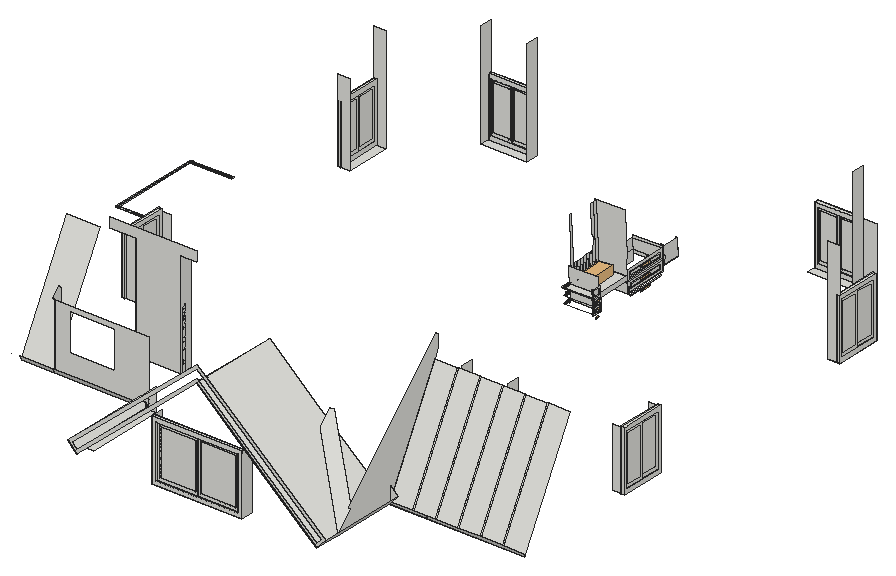
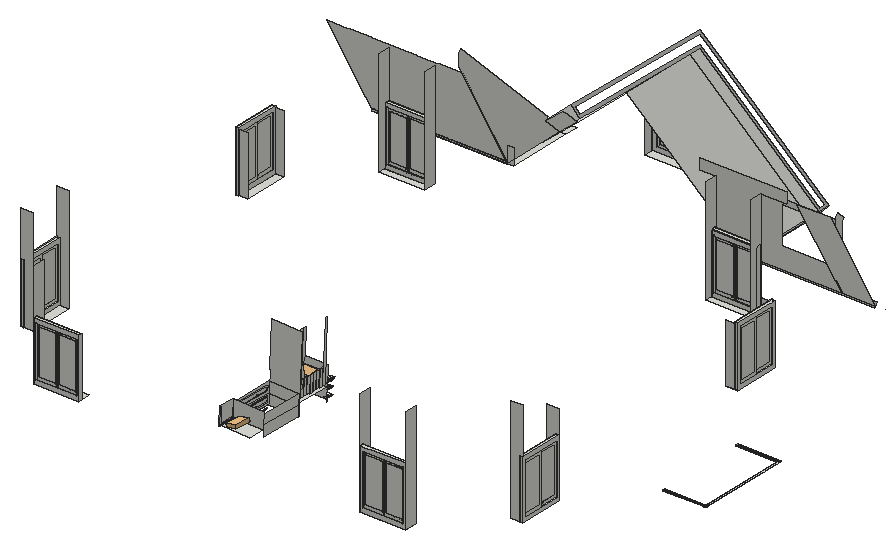
# SketchUp Ruby script. Lengths in inches.
U = 1.inch
M = Sketchup.active_model
def pt(a) = Geom::Point3d.new(a.map { |v| v * U })
def face(e, loops, mat)
  f = e.add_face(loops[0].map { |a| pt(a) })
  loops[1..].each { |l| e.add_face(l.map { |a| pt(a) }).erase! }
  f.material = f.back_material = mat if mat
  f
end
# faces: each face lists its corners as indices into pts; further lists are holes
def faces(e, pts, list, mat = nil) = list.each { |f| face(e, (f[0].is_a?(Array) ? f : [f]).map { |l| l.map { |i| pts[i] } }, mat) }
# xy, xz, yz: faces in a plane at the given z, y or x. An outline is a flat list of corners, or four numbers for a rectangle; further outlines are holes
def ring(l) = l.size == 4 ? [[l[0], l[1]], [l[2], l[1]], [l[2], l[3]], [l[0], l[3]]] : l.each_slice(2).to_a
def flat(e, list, mat, &to3) = list.each { |f| face(e, (f[0].is_a?(Array) ? f : [f]).map { |l| ring(l).map { |u, v| to3.(u, v) } }, mat) }
def xy(e, z, list, mat = nil) = flat(e, list, mat) { |x, y| [x, y, z] }
def xz(e, y, list, mat = nil) = flat(e, list, mat) { |x, z| [x, y, z] }
def yz(e, x, list, mat = nil) = flat(e, list, mat) { |y, z| [x, y, z] }
def lines(e, pts, list) = list.each { |a, b| e.add_line(pt(pts[a]), pt(pts[b])) }
# prism: a flat outline (further loops are holes) pulled along v
def prism(e, loops, v, mat = nil)
  f = face(e, loops, mat); d = Geom::Vector3d.new(v.map { |x| x * U })
  f.pushpull(f.normal.samedirection?(d) ? d.length : -d.length)
end
def box(e, o, s, mat = nil) = prism(e, [[o, [o[0] + s[0], o[1], o[2]], [o[0] + s[0], o[1] + s[1], o[2]], [o[0], o[1] + s[1], o[2]]]], [0, 0, s[2]], mat)
def at(x, y, z, deg = 0) = Geom::Transformation.translation(pt([x, y, z])) * Geom::Transformation.rotation(ORIGIN, Z_AXIS, deg.degrees)
def axes(o, x, y, z) = Geom::Transformation.new([*x, 0, *y, 0, *z, 0, *pt(o).to_a, 1])
def part(name) = M.definitions.add(name)
# library, detail: a bought-in or finely detailed component or shape, given as its bounding box
def library(name, o, s) = part(name).tap { |d| box(d.entities, o, s) }
def detail(e, o, s) = box(e.add_group.entities, o, s)
def put(e, d, t, mat = nil) = e.add_instance(d, t).tap { |i| i.material = mat if mat }
def group(e, t, mat = nil) = e.add_group.tap { |g| g.transformation = t; g.material = mat if mat }.entities
root = M.entities
c1 = library("Group\#35",[0,0,0],[1.97,1.34,1.72])
c2 = library("Group\#46",[0,0,0],[1.97,1.34,1.72])
c3 = library("Agrupar\#1",[0,0,0],[17.89,11.02,4.2])
c4 = library("Group\#28",[0,0,0],[1.97,1.34,1.72])
c5 = part("Group691\#1")
box(c5.entities,[-2739.57,269.12,161.53],[33.66,1.73,0.47])
c6 = part("Group695\#1")
box(c6.entities,[-2739.57,196.24,161.53],[33.66,1.73,0.47])
c7 = part("Group699\#1")
box(c7.entities,[-2740.2,196.87,161.53],[1.73,73.35,0.47])
c8 = part("Sliding window")
xy(c8.entities,0,[[0,0,4.33,55.51]])
xy(c8.entities,2.76,[[0,2.76,2,27.76],[3.15,2.76,4.33,27.76],[0,27.76,0.82,52.76],[0.82,27.76,2.36,52.76],[2.36,27.76,4.33,52.76]])
xy(c8.entities,4.72,[[2,4.72,2.4,26.38],[2.76,4.72,3.15,26.38],[0.82,29.13,1.22,50.79],[1.97,29.13,2.36,50.79]])
xy(c8.entities,36.61,[[2,4.72,2.4,26.38],[2.76,4.72,3.15,26.38],[0.82,29.13,1.22,50.79],[1.97,29.13,2.36,50.79]])
xy(c8.entities,38.58,[[0,2.76,2,27.76],[3.15,2.76,4.33,27.76],[0,27.76,0.82,52.76],[0.82,27.76,2.36,52.76],[2.36,27.76,4.33,52.76]])
xy(c8.entities,41.34,[[0,0,4.33,55.51]])
xz(c8.entities,0,[[0,0,4.33,41.34]])
xz(c8.entities,2.76,[[0,2.76,2,38.58],[3.15,2.76,4.33,38.58]])
xz(c8.entities,4.72,[[2,4.72,2.4,36.61],[2.76,4.72,3.15,36.61]])
xz(c8.entities,26.38,[[2,4.72,2.4,36.61],[2.76,4.72,3.15,36.61]])
xz(c8.entities,27.76,[[0.82,2.76,2,38.58],[2,2.76,2.36,38.58],[2.36,2.76,3.15,38.58]])
xz(c8.entities,29.13,[[0.82,4.72,1.22,36.61],[1.97,4.72,2.36,36.61]])
xz(c8.entities,50.79,[[0.82,4.72,1.22,36.61],[1.97,4.72,2.36,36.61]])
xz(c8.entities,52.76,[[0,2.76,0.82,38.58],[0.82,2.76,2.36,38.58],[2.36,2.76,4.33,38.58]])
xz(c8.entities,55.51,[[0,0,4.33,41.34]])
yz(c8.entities,0,[[[0,0,55.51,41.34],[2.76,2.76,52.76,38.58]]])
yz(c8.entities,0.82,[[[27.76,2.76,52.76,38.58],[29.13,4.72,50.79,36.61]]])
yz(c8.entities,1.22,[[29.13,4.72,50.79,36.61]])
yz(c8.entities,1.97,[[29.13,4.72,50.79,36.61]])
yz(c8.entities,2,[[[2.76,2.76,27.76,38.58],[4.72,4.72,26.38,36.61]]])
yz(c8.entities,2.36,[[[27.76,2.76,52.76,38.58],[29.13,4.72,50.79,36.61]]])
yz(c8.entities,2.4,[[4.72,4.72,26.38,36.61]])
yz(c8.entities,2.76,[[4.72,4.72,26.38,36.61]])
yz(c8.entities,3.15,[[[2.76,2.76,27.76,38.58],[4.72,4.72,26.38,36.61]]])
yz(c8.entities,4.33,[[[0,0,55.51,41.34],[2.76,2.76,52.76,38.58]]])
c9 = library("Linha+BT+Oruy+porta+maquiagem+suporte+batom+espelho+de+mão+c",[21.99,11.32,0],[36.15,16.65,11.83])
xy(root,162,[[185.113,1.565,185.113,71.567,185.069,71.567],[245,1.565,317,11.565],[185.113,11.565,191,73.565],[371,11.565,376.6875,21.7],[371,21.7,376.6875,73.565],
  [185.068,71.567,185.069,71.567,185.068,73.565],[185.069,71.567,185.113,71.567,185.113,73.565,185.068,73.565],[136,121.565,172,131.565],[396,121.565,432,131.565],[474,173.565,484,209.565],
  [84,387.565,94,423.565],[474,387.565,484,423.565],[136,465.565,172,475.565],[396,465.565,432,475.565]])
xy(root,162.6875,[[84,173.565,94,209.565]])
xz(root,1.565,[[[185.113,162,191,167.157,245,214.457,281.011,246,317.023,214.383,371,166.993,376.6875,162,383.285,169.515,281.019,259.3,178.524,169.522,183.854,163.437],[185.31,164.988,181.511,169.325,281.017,256.485,380.297,169.321,376.493,164.988,372.397,168.584,318.42,215.974,281.013,248.816,243.605,216.049,189.605,168.749]]])
xz(root,73.565,[[185.113,162,185.068,162.051,185.113,163.437],[185.113,162,191,162,191,167.157],[185.113,162,191,167.157,191,180.451,185.113,175.294],[371,162,371,166.993,376.6875,162],[376.6875,162,371,166.993,371,175.307,376.6875,175.307],
  [376.6875,162,376.6875,163.437,377.949,163.437],[377.949,162,484.068,163.437],[185.068,162.051,185.068,163.479,178.524,169.522,183.854,163.437],[185.068,162.051,185.068,163.437,185.113,163.437],[[110,163.437,183.854,163.437,178.524,169.522,185.068,175.254,185.068,214,110,214],[122,180,158,210]],
  [185.068,163.437,185.113,163.437,185.068,163.479,178.524,169.522,185.068,175.254],[185.068,163.437,185.068,163.479,185.113,163.437],[185.113,163.437,185.068,163.479,185.068,175.254,185.113,175.294],[376.6875,163.437,376.6875,175.307,383.285,169.515,377.949,163.437]])
xz(root,121.565,[[136,162,136,246,116,246,116,254.0625,185.113,254.0625,185.113,246,172,246,172,162]])
xz(root,173.565,[[474,162,484,209.3125],[84,162.6875,94,209.3125]])
xz(root,209.565,[[474,162,484,209.3125],[84,162.6875,94,209.3125]])
xz(root,387.565,[[84,162,94,227.656],[474,162,484,246]])
xz(root,423.565,[[84,162,94,246],[474,162,484,246]])
yz(root,110,[[73.565,163.437,73.565,214,71.662,215.898,71.733,215.969,73.636,214.071,73.636,163.567],[73.636,163.567,73.636,214.071,71.733,215.969,77.662,221.914,79.565,220.016,79.565,174.507]])
yz(root,136,[[121.565,162,131.565,246],[465.565,162,475.565,246]])
yz(root,172,[[121.565,162,131.565,246],[465.565,162,475.565,246]])
yz(root,245,[[1.565,162,11.565,210]])
yz(root,317,[[1.565,162,11.565,210]])
yz(root,376.6875,[[21.7,162,73.565,162,73.565,163.437,118.313,246,121.565,252,121.565,262.125,119.662,264.023,33.07,177.205,34.973,175.307]])
yz(root,396,[[121.565,162,131.565,246]])
yz(root,432,[[121.565,162,131.565,246],[465.565,162,475.565,246]])
p = [[313.457,392.262,148.566],[313.457,420.995,149.218],[313.654,420.995,149.223],[313.654,392.262,148.571],[290.161,361.337,148.842],[290.212,361.337,148.843],
  [290.108,361.283,151.203],[313.451,421.664,149.516],[313.451,391.974,148.842],[313.648,391.974,148.846],[313.648,421.664,149.52],[313.645,391.859,148.955],
  [313.645,421.773,149.634],[313.636,422.158,150.037],[313.636,391.457,149.34],[313.448,391.86,148.951],[313.448,393.434,148.987],[313.448,421.773,149.63],
  [313.457,421.388,149.227],[313.654,421.388,149.232],[313.579,388.87,159.226],[289.963,388.882,158.69],[290.153,389.072,150.328],[313.769,389.06,150.864],
  [313.6,389.847,150.878],[290.153,389.859,150.346],[289.963,389.669,158.708],[313.411,389.657,159.24],[313.532,389.779,153.877],[313.566,389.813,152.377],
  [313.581,389.827,151.74],[313.75,389.827,151.743],[313.753,389.831,151.582],[313.76,389.838,151.275],[313.769,389.847,150.882],[290.153,423.708,151.114],
  [289.963,423.519,159.476],[313.758,354.618,150.559],[313.758,361.031,150.705],[314.619,361.031,150.724],[314.619,354.617,150.579],[313.61,361.058,157.249],
  [313.547,360.996,160.003],[290.24,361.008,159.475],[290.629,361.208,150.641],[313.748,361.196,151.166],[313.744,361.192,151.347],[313.614,361.0625,157.068],
  [313.769,423.696,151.65],[313.76,423.6875,152.044],[313.751,423.678,152.437],[313.75,423.677,152.512],[313.769,421.484,151.6],[314.605,354.515,151.215],
  [314.609,354.519,151.034],[313.748,354.519,151.014],[313.744,354.515,151.195],[313.744,361.167,151.346],[313.744,354.867,151.203],[313.744,354.54,151.196],
  [313.748,354.544,151.015],[313.748,361.172,151.165],[314.609,354.544,151.034],[314.609,361.171,151.185],[290.108,356.892,151.114],[290.108,355.97,151.093],
  [292.095,355.969,151.138],[292.095,356.891,151.159],[290.108,358.737,151.156],[290.108,357.815,151.135],[292.095,357.813,151.18],[292.095,358.736,151.201],
  [314.475,354.385,156.936],[313.614,354.385,156.917],[313.614,354.41,156.917],[314.605,354.54,151.215],[314.605,361.167,151.366],[314.475,361.037,157.087],
  [314.475,354.41,156.937],[314.485,360.985,156.629],[314.594,361.094,151.821],[314.594,354.592,151.674],[314.485,354.483,156.481],[314.485,360.897,156.627],
  [314.609,361.196,151.185],[313.759,361.196,151.166],[313.755,361.192,151.347],[314.605,361.192,151.366],[313.614,361.038,157.068],[313.625,361.0625,157.068],
  [314.475,361.062,157.088],[313.581,423.677,152.508],[313.411,423.507,160.008],[313.411,421.295,159.958],[313.584,389.831,151.578],[313.591,389.838,151.272],
  [313.591,423.6875,152.04],[313.446,421.968,158.398],[313.549,422.071,153.859],[313.549,391.37,153.163],[313.446,391.267,157.702],[313.724,354.476,151.584],
  [313.725,355.116,151.599],[313.725,354.476,151.584],[290.097,359.988,151.643],[290.097,359.201,151.625],[292.065,359.2,151.67],[292.065,359.987,151.6875],
  [313.624,354.484,156.462],[313.733,354.593,151.654],[313.733,361.094,151.802],[313.624,360.985,156.609],[313.624,360.897,156.607],[313.356,423.677,152.503],
  [313.356,389.827,151.734],[313.735,389.8125,152.381],[290.09,359.981,151.961],[290.09,359.194,151.943],[292.058,359.193,151.987],[292.058,359.98,152.005],
  [290.09,361.556,151.996],[290.09,360.768,151.979],[292.058,360.767,152.023],[292.058,361.555,152.041],[313.701,389.779,153.88],[313.579,423.507,160.012],
  [313.54,391.755,153.565],[313.455,391.67,157.317],[313.54,421.668,154.244],[313.344,421.668,154.24],[313.258,421.583,157.992],[313.258,393.244,157.348],
  [313.258,391.67,157.3125],[313.344,391.755,153.561],[313.341,421.554,154.349],[313.341,391.864,153.675],[313.261,391.784,157.204],[313.261,421.474,157.877],
  [313.538,391.864,153.679],[313.458,391.784,157.208],[313.538,421.554,154.353],[313.458,421.474,157.882],[313.464,421.199,157.594],[313.531,421.266,154.629],
  [313.531,392.14,153.968],[313.464,392.072,156.933],[313.464,420.805,157.585],[313.579,389.657,159.244],[313.455,421.583,157.996],[313.267,392.072,156.928],
  [313.335,392.14,153.963],[313.335,421.266,154.624],[313.267,421.199,157.589],[313.267,420.805,157.58],[313.664,437.367,156.586],[313.646,437.349,157.373],
  [313.646,424.361,157.079],[313.664,424.379,156.292],[314.845,424.378,156.318],[314.827,424.36,157.105],[314.845,437.367,156.613],[314.827,437.349,157.4],
  [290.03,424.373,156.543],[289.736,424.078,169.528],[313.352,424.066,170.064],[290.03,437.362,156.838],[289.978,356.763,156.82],[289.978,355.84,156.799],
  [291.966,355.839,156.844],[291.966,356.762,156.865],[289.978,358.607,156.862],[289.978,357.685,156.841],[291.966,357.684,156.886],[291.966,358.606,156.907],
  [313.494,360.942,162.364],[313.476,360.924,163.151],[313.476,354.599,163.008],[313.476,354.247,163],[313.494,354.265,162.213],[313.61,354.381,157.098],
  [313.61,354.733,157.106],[313.61,354.406,157.098],[313.494,354.29,162.213],[313.48,354.276,162.82],[313.48,360.904,162.97],[313.494,360.917,162.364],
  [313.61,361.033,157.249],[314.471,354.381,157.117],[314.337,354.247,163.019],[314.471,354.406,157.118],[314.471,361.033,157.268],[314.341,360.903,162.989],
  [314.341,354.276,162.839],[314.351,360.851,162.531],[314.46,360.96,157.724],[314.46,354.458,157.576],[314.351,354.349,162.383],[314.351,360.763,162.529],
  [313.621,361.058,157.249],[314.471,361.058,157.269],[314.532,424.065,170.091],[314.532,437.054,170.386],[313.487,360.924,163.152],[314.337,360.924,163.171],
  [289.968,359.859,157.349],[289.968,359.072,157.331],[291.936,359.071,157.375],[291.936,359.858,157.393],[313.352,437.055,170.359],[313.59,354.343,157.487],
  [313.591,354.982,157.501],[313.591,354.343,157.487],[313.494,354.353,162.215],[313.49,354.35,162.364],[313.599,354.459,157.557],[313.599,360.96,157.704],
  [313.494,360.854,162.362],[313.49,360.851,162.511],[289.956,358.273,157.827],[289.956,357.486,157.809],[291.924,357.485,157.854],[291.924,358.272,157.872],
  [289.956,359.847,157.863],[289.956,359.06,157.845],[291.924,359.059,157.89],[291.924,359.846,157.908],[313.547,388.838,160.635],[289.931,388.85,160.099],
  [289.774,423.329,167.838],[289.774,389.479,167.07],[313.221,389.467,167.602],[313.342,389.589,162.238],[313.376,389.623,160.739],[313.391,389.637,160.101],
  [313.56,389.637,160.105],[313.563,389.641,159.944],[313.57,389.648,159.637],[313.57,423.498,160.405],[313.561,423.489,160.799],[313.56,423.487,160.873],
  [313.579,421.294,159.962],[290.124,360.948,162.125],[289.982,361.008,159.469],[289.931,361.008,159.468],[313.391,423.487,160.87],[313.221,423.317,168.37],
  [313.221,421.105,168.32],[313.395,389.641,159.94],[313.402,389.648,159.633],[313.402,423.498,160.402],[313.256,421.778,166.76],[313.359,421.881,162.221],
  [313.359,391.18,161.525],[313.256,391.077,166.064],[313.476,388.766,163.783],[289.86,388.778,163.247],[291.828,388.777,163.292],[313.166,423.487,160.864],
  [313.166,389.638,160.096],[313.545,389.623,160.743],[313.511,389.589,162.242],[313.389,423.317,168.374],[313.351,391.565,161.927],[313.265,391.48,165.679],
  [313.351,421.479,162.606],[289.584,377.482,175.164],[289.584,375.907,175.128],[289.86,376.183,162.962],[289.89,376.214,161.617],[289.89,377.788,161.653],
  [289.86,377.758,162.997],[291.858,376.213,161.662],[291.828,376.182,163.006],[291.858,377.787,161.697],[291.828,377.757,163.042],[291.828,376.97,163.024],
  [288.78,364.083,210.293],[288.78,362.508,210.257],[289.86,363.588,162.676],[289.877,363.605,161.941],[289.877,365.179,161.977],[289.86,365.163,162.712],
  [291.845,365.178,162.021],[291.845,363.604,161.985],[291.828,363.587,162.72],[313.154,391.565,161.923],[313.069,391.48,165.675],[313.154,421.479,162.601],
  [313.069,421.394,166.353],[313.069,393.054,165.71],[313.151,421.365,162.71],[313.151,391.674,162.037],[313.071,391.594,165.565],[313.071,421.285,166.239],
  [183.854,1.565,163.437],[183.854,73.565,163.437],[185.068,73.565,162.051],[185.113,73.565,162],[185.113,71.567,162],[185.113,11.565,162],
  [185.113,1.565,162],[245,1.565,214.457],[191,1.565,167.157],[281.011,11.565,246],[281.011,1.565,246],[371,1.565,166.993],
  [317.023,1.565,214.383],[376.6875,11.565,162],[376.6875,1.565,162],[376.6875,21.7,162],[376.6875,73.565,162],[377.949,73.565,163.437],
  [383.285,73.565,169.515],[383.285,1.565,169.515],[191,73.565,167.157],[191.068,73.565,167.216],[244.479,73.565,214],[281.011,73.565,246],
  [317.459,73.565,214],[371,73.565,166.993],[376.6875,34.973,175.307],[371,39.953,180.301],[332.616,73.565,214],[329.3125,73.565,214],
  [329.3125,63.186,203.593],[185.068,73.565,162],[110,73.636,162],[109.999,72.07,165.13],[132.596,72.048,165.13],[150.478,72.032,165.13],
  [168.361,72.015,165.13],[185.066,72,165.13],[484.068,73.565,162],[407.25,73.636,162],[407.249,72.07,165.13],[413.713,72.065,165.13],
  [431.596,72.048,165.13],[449.478,72.032,165.13],[467.361,72.015,165.13],[484.066,72,165.13],[83.984,73.66,162],[83.983,72.095,165.13],
  [376.773,73.658,161.997],[376.771,72.093,165.127],[395.831,72.079,165.129],[289.871,354.697,162.003],[291.828,354.928,162.524],[291.828,355.715,162.542],
  [289.871,355.619,162.024],[289.871,356.541,162.045],[291.828,356.502,162.56],[291.828,357.29,162.578],[289.871,357.463,162.066],[291.828,365.162,162.756],
  [291.828,364.374,162.738],[291.828,363.591,162.72],[313.348,391.674,162.041],[313.268,391.594,165.57],[313.348,421.365,162.715],[313.268,421.284,166.244],
  [313.274,421.009,165.955],[313.342,421.076,162.99],[313.342,391.95,162.329],[313.274,391.882,165.294],[313.274,420.615,165.946],[289.584,360.66,174.782],
  [289.602,360.678,173.995],[289.705,360.732,171.635],[313.342,360.79,169.054],[313.338,360.786,169.235],[312.477,360.787,169.215],[312.347,360.657,174.936],
  [312.428,360.657,174.938],[312.419,360.649,175.3],[291.552,360.659,174.827],[291.346,360.66,174.822],[289.584,368.035,174.949],[289.584,366.461,174.914],
  [289.86,366.737,162.747],[289.874,366.752,162.103],[289.874,368.326,162.139],[289.86,368.311,162.783],[291.842,366.751,162.148],[291.828,366.736,162.792],
  [291.842,368.325,162.183],[291.828,368.31,162.828],[291.828,367.523,162.81],[313.494,354.147,162.21],[313.476,354.13,162.997],[313.49,360.763,162.509],
  [313.389,389.467,167.606],[313.265,421.393,166.358],[313.145,391.95,162.325],[313.078,391.883,165.29],[313.145,421.076,162.986],[313.078,421.009,165.951],
  [313.078,420.615,165.942],[289.86,358.078,162.551],[291.828,358.077,162.595],[291.828,354.141,162.506],[291.828,387.203,163.256],[291.828,386.416,163.238],
  [291.828,385.629,163.221],[291.828,385.625,163.221],[291.828,384.054,163.185],[291.828,384.051,163.185],[291.828,383.267,163.167],[291.828,382.48,163.149],
  [291.828,381.693,163.131],[291.828,380.905,163.113],[291.828,380.118,163.096],[291.828,379.331,163.078],[291.828,378.544,163.06],[291.828,375.395,162.988],
  [291.828,374.608,162.971],[291.828,373.821,162.953],[291.828,373.034,162.935],[291.828,372.246,162.917],[291.828,371.459,162.899],[291.828,370.672,162.881],
  [291.828,369.885,162.863],[291.828,369.098,162.845],[291.828,365.949,162.774],[291.828,362.8,162.703],[291.828,362.013,162.685],[291.828,361.226,162.667],
  [291.828,360.438,162.649],[291.828,359.651,162.631],[291.828,358.864,162.613],[289.86,358.865,162.569],[289.584,371.184,175.021],[289.584,369.61,174.985],
  [289.86,369.886,162.819],[289.866,369.892,162.548],[289.866,371.466,162.584],[289.86,371.46,162.854],[291.834,369.891,162.593],[291.834,371.465,162.629],
  [289.86,359.652,162.586],[289.86,360.439,162.604],[289.86,361.227,162.622],[289.86,362.014,162.64],[289.86,362.801,162.658],[291.592,364.926,173.14],
  [291.569,363.329,174.114],[289.86,364.375,162.694],[289.86,365.95,162.729],[291.623,368.105,171.869],[291.611,366.519,172.336],[289.86,367.524,162.765],
  [289.86,369.099,162.801],[289.86,370.673,162.837],[289.584,374.333,175.092],[289.584,372.758,175.057],[289.86,373.035,162.89],[289.862,373.036,162.805],
  [289.862,374.611,162.841],[289.86,374.609,162.926],[291.83,374.61,162.886],[291.83,373.035,162.85],[289.864,378.549,162.849],[289.86,378.545,163.015],
  [291.832,378.548,162.894],[291.632,371.263,171.53],[291.63,369.687,171.568],[289.86,372.247,162.872],[291.623,374.403,172.014],[291.63,372.836,171.635],
  [289.86,373.822,162.908],[289.86,375.396,162.944],[289.584,380.63,175.235],[289.584,379.056,175.199],[289.86,379.332,163.033],[289.863,379.335,162.903],
  [289.863,380.909,162.939],[289.86,380.907,163.069],[291.831,379.334,162.948],[291.831,380.908,162.984],[314.199,354.109,169.103],[313.338,354.109,169.083],
  [313.472,354.268,163.181],[313.342,354.138,168.903],[313.338,354.134,169.084],[313.342,360.766,169.053],[313.472,360.895,163.332],[291.593,377.522,173.403],
  [291.611,375.966,172.555],[289.86,376.971,162.979],[291.552,380.629,175.28],[291.534,380.612,176.062],[291.535,380.589,176.025],[291.567,379.07,174.579],
  [289.86,380.119,163.051],[289.856,380.116,163.217],[291.824,380.115,163.262],[289.86,384.052,163.14],[289.86,383.268,163.122],[289.858,383.266,163.22],
  [289.856,383.264,163.288],[291.824,383.263,163.333],[291.826,383.265,163.264],[289.86,384.055,163.14],[289.832,354.773,163.194],[289.832,353.85,163.174],
  [291.82,353.849,163.219],[291.82,354.772,163.24],[314.333,354.268,163.201],[314.333,360.895,163.351],[314.203,360.765,169.073],[314.203,354.138,168.922],
  [314.213,360.713,168.614],[314.322,360.822,163.807],[314.322,354.32,163.659],[314.213,354.211,168.467],[314.213,360.625,168.612],[289.832,356.617,163.236],
  [289.832,355.695,163.215],[291.82,355.694,163.26],[291.82,356.616,163.281],[313.349,360.786,169.235],[314.199,360.786,169.254],[290.748,381.4,210.73],
  [291.233,381.886,189.335],[291.259,382.498,188.213],[291.331,383.255,185.083],[291.404,383.176,181.863],[291.473,382.267,178.774],[291.478,382.13,178.55],
  [291.552,382.204,175.316],[291.826,382.478,163.246],[291.826,384.052,163.282],[291.552,383.778,175.351],[290.748,382.975,210.766],[290.748,382.581,210.757],
  [290.748,382.1875,210.748],[289.584,382.205,175.271],[289.858,382.479,163.202],[289.584,383.779,175.307],[289.858,384.053,163.237],[291.552,386.927,175.423],
  [290.748,386.123,210.838],[290.748,385.73,210.829],[290.748,385.336,210.82],[290.748,384.549,210.802],[291.552,385.353,175.387],[289.584,386.928,175.378],
  [289.584,385.354,175.342],[289.86,385.63,163.176],[289.86,386.417,163.194],[289.86,387.204,163.212],[289.86,385.626,163.176],[289.584,388.502,175.414],
  [289.774,388.692,167.052],[313.389,388.68,167.588],[313.381,388.671,167.981],[313.212,388.671,167.977],[313.205,388.664,168.284],[313.201,388.661,168.445],
  [312.976,388.661,168.44],[312.962,388.646,169.078],[312.928,388.612,170.577],[312.878,388.562,172.793],[312.806,388.49,175.941],[313.2,388.49,175.95],
  [312.396,387.687,211.364],[288.78,387.699,210.829],[289.832,358.462,163.278],[289.832,357.539,163.257],[291.82,357.538,163.302],[291.82,358.461,163.323],
  [178.524,73.565,169.522],[178.524,1.565,169.522],[110,73.565,163.437],[110,73.636,163.567],[110,79.565,174.507],[110,118.313,246],
  [84,118.313,246],[84,73.565,163.437],[376.6875,73.565,163.437],[483.993,73.636,163.567],[483.993,79.565,174.507],[484.1875,118.313,246],
  [484.084,118.313,246],[484,118.313,246],[467.479,118.313,246.001],[466.302,118.313,246],[449.594,118.313,246.001],[448.417,118.313,246],
  [431.708,118.313,246.001],[430.531,118.313,246],[413.823,118.313,246.001],[412.646,118.313,246],[395.9375,118.313,246.001],[394.76,118.313,246],
  [376.875,118.313,246],[376.6875,118.313,246],[484.068,73.565,163.437],[313.456,354.209,163.389],[313.457,354.848,163.404],[313.457,354.209,163.389],
  [313.352,354.212,168.447],[313.461,354.321,163.64],[313.461,360.822,163.787],[313.352,360.713,168.595],[313.352,360.625,168.593],[289.822,359.713,163.765],
  [289.822,358.926,163.747],[291.79,358.925,163.792],[291.79,359.712,163.81],[75.5,73.565,163.541],[75.5,73.565,163.437],[313.642,410.103,155.861],
  [313.641,410.102,155.9],[313.601,354.343,157.487],[313.6,421.484,151.596],[289.974,361.15,157.105],[290.027,361.203,154.744],[313.691,402.687,155.746],
  [313.692,402.688,155.747],[313.831,410.292,147.499],[313.831,410.445,147.502],[313.186,421.295,159.953],[290.078,361.203,154.745],[313.375,421.484,151.591],
  [313.714,409.965,147.656],[313.714,410.026,147.658],[313.661,409.972,147.428],[313.71,409.983,147.599],[313.727,403.694,147.216],[313.723,403.69,147.386],
  [313.516,402.473,155.721],[313.521,402.655,155.719],[313.881,402.877,147.384],[313.881,402.878,147.385],[289.974,354.355,156.951],[313.514,402.649,155.69],
  [313.642,410.255,155.864],[313.718,410.03,147.501],[313.83,410.292,147.538],[289.86,382.481,163.105],[291.824,381.689,163.297],[289.856,386.413,163.36],
  [291.824,386.412,163.405],[289.856,381.69,163.253],[289.86,381.694,163.087],[289.822,360.5,163.783],[313.467,354.209,163.389],[289.974,358.796,157.052],
  [289.956,360.634,157.881],[291.924,360.633,157.926],[290.108,354.489,151.049],[289.944,361.069,160.648],[289.893,361.069,160.646],[289.84,354.221,162.853],
  [289.956,361.422,157.899],[291.79,360.499,163.828],[290.09,358.407,151.925],[292.058,358.406,151.97],[290.103,358.925,151.346],[289.972,358.867,157.124],
  [290.102,358.996,151.418],[313.735,354.476,151.585],[289.951,361.077,160.314],[289.901,361.077,160.313],[290.108,355.048,151.072],[292.095,355.047,151.117],
  [289.978,354.918,156.778],[290.081,361.206,154.608],[290.03,361.206,154.607],[290.097,360.776,151.661],[292.065,360.775,151.705],[289.968,360.646,157.367],
  [291.936,360.645,157.411],[290.215,361.34,148.712],[290.164,361.34,148.711],[292.058,357.619,151.952],[290.09,356.832,151.889],[291.966,354.917,156.823],
  [466.198,73.47,163.437],[466.198,118.218,246],[394.657,73.47,163.437],[394.657,118.218,246],[412.542,73.47,163.437],[412.542,118.218,246],
  [376.771,73.47,163.437],[376.771,118.218,246],[430.427,73.47,163.437],[430.427,118.218,246],[448.313,73.47,163.437],[448.313,118.218,246],
  [449.49,73.47,163.4375],[449.49,118.218,246.001],[467.375,73.47,163.4375],[467.375,118.218,246.001],[395.834,73.47,163.4375],[395.834,118.218,246.001],
  [413.719,73.47,163.4375],[413.719,118.218,246.001],[431.604,73.47,163.4375],[431.604,118.218,246.001],[313.472,409.782,155.79],[313.52,409.793,155.961],
  [313.452,409.913,164.223],[313.451,409.912,164.262],[313.334,409.585,164.38],[313.334,409.646,164.382],[313.524,409.836,156.02],[313.528,409.84,155.863],
  [313.537,403.504,155.578],[313.533,403.5,155.748],[313.452,410.065,164.226],[313.347,403.314,163.939],[313.344,403.31,164.11],[313.282,409.593,164.152],
  [313.33,409.603,164.323],[313.338,409.651,164.225],[313.524,409.775,156.018],[313.501,402.497,164.108],[313.502,402.499,164.109]]
faces(root,p,[[0,1,2,3],[4,5,6],[7,8,9,10],[11,12,13,14],[12,11,15,16,17],[1,18,19,2],[20,21,22,23],[24,25,26,27,28,29,30,31,32,33,34],
  [25,35,36,26],[37,38,39,40],[41,42,43,44,45,46,47],[48,49,50,51,31,32,33,34,52],[53,54,55,56],[45,46,57,58,59,56,55,60,61],[54,62,60,55],[61,60,62,63],
  [64,65,66,67],[68,69,70,71],[72,53,56,73],[73,56,59,74],[[75,76,77,78],[79,80,81,82,83]],[56,59,75,53],[59,58,57,76,75],[45,61,63,84,85],
  [85,86,46,45],[84,87,86,85],[88,57,46,47],[57,88,77,76],[47,46,86,89],[89,86,87,90],[87,76,57,46,86],[[91,92,93,27,28,29,30,94,95,96],[97,98,99,100]],
  [101,102,103],[104,105,106,107],[108,109,110,111,112],[109,108,82,81],[110,109,81,80],[31,51,91,113,114,30],[31,30,29,115],[111,110,80,79],
  [116,117,118,119],[120,121,122,123],[115,29,28,124],[125,92,91,51],[100,99,126,127],[99,98,128,126],[[129,130,131,132,133],[134,135,136,137]],[127,126,133,132],
  [126,128,129,133],[136,135,138,139],[[138,140,141,139],[142,143,144,145,146]],[135,134,140,138],[27,147,124,28],[148,128,98,97],[149,150,151,152,153],[150,149,145,144],
  [151,150,144,143],[128,148,130,129],[134,137,141,140],[152,151,143,142],[154,155,156,157],[158,159,156,157],[154,157,158,160],[160,161,159,158],
  [108,112,83,82],[162,163,164,156],[155,165,162,156],[161,160,154,155],[166,167,168,169],[170,171,172,173],[[47,41,42,174,175,176,177,178,179,73,74,88],[180,181,182,183,184,185,186]],[72,78,74,73],
  [74,88,47,41,186,180,181,179,73],[187,72,73,179],[88,74,78,77],[149,153,146,145],[188,187,179,178,177],[[189,190,191,192],[193,194,195,196,197]],[179,181,189,187],[181,180,186,190,189],
  [47,88,77,90,89],[41,47,89,198],[90,199,198,89],[164,156,159,200],[200,159,161,201],[156,155,161,159],[186,185,184,191,190],[42,174,185,186,41],
  [198,202,175,174,42,41],[202,198,199,203],[199,190,186,41,198],[137,136,139,141],[204,205,206,207],[127,148,97,100],[148,127,132,131,130],[155,208,201,161],
  [209,210,211],[212,213,196,195,214],[215,216,212,214],[215,214,195,194],[153,152,142,146],[217,216,215,194,193],[218,219,220,221],[222,223,224,225],
  [20,226,227,21],[26,36,228,229],[27,26,229,230,231,232,233,234,235,236,147],[125,237,238,239,234,235,236,147,240],[241,43,42,174,175],[226,42,43,242,243,227],[238,239,244,245,228,36,92,125,237],[[244,245,246,230,231,232,233,247,248,249],[250,251,252,253]],
  [254,175,174,42,226],[255,227,226,254,256],[234,239,244,257,258,233],[234,233,232,259],[259,232,231,260],[261,245,244,239],[253,252,262,263],[252,251,264,262],
  [265,266,267,268,269,270],[271,272,267,268],[269,273,271,268],[273,274,275,272,271],[269,270,274,273],[276,277,278,279,280,281],[282,283,279,280],[284,278,279,283],
  [263,262,285,286],[[287,288,289,286,285],[290,291,292,293]],[262,264,287,285],[294,295,296,297,298,299,300],[301,302,300,299,303,304],[305,306,304,303,307,308],[308,307,309,310,311,312,313],[303,299,298,297,314,315,316,317],
  [307,303,317,318,319,310,309],[309,320,321,322,323,324],[325,326,327,328,329,330,331],[332,333,334,335,336,337,338,339],[326,340,341,327],[333,342,343,344,334],[345,346,347,348],[349,350,351,352],
  [282,353,354,355,284,283],[280,281,353,282],[292,291,356,357],[[356,358,359,357],[360,361,362,363,364]],[291,290,358,356],[365,366,367,241,175,368,369,370,371,372,373,374,375],[376,377,378,379,380,381],[382,383,378,379],
  [384,385,386,383,382],[380,384,382,379],[380,381,385,384],[387,178,177,388],[178,182,183,184,185,174,175,176,177],[216,185,184,183,182,212,213,389,217],[212,216,217,389,213],[230,390,260,231],
  [391,264,251,250],[392,393,363,362],[394,392,362,361],[393,392,394,395,396],[213,389,197,196],[397,398,351,350,347,346,399,388,177,176,175,254,256,400,401,402,403,404,405,406,407,408,409,410,411,412,274,275,272,413,414,415,416,417,418,419,420,421,385,386,383,422,353,354,355,284,423,424,425,426,427,428,429],[430,431,432,433,434,435],[436,433,434,437],
  [436,420,432,433],[438,427,426,439],[440,425,424,441],[437,418,419,420,436],[434,435,418,437],[264,391,288,287],[423,284,278,442],[353,443,444,284,355,354],
  [355,278,284],[445,354,353,281],[446,422,383,378],[290,293,359,358],[184,183,192,191],[385,447,448,383,386],[449,386,385,381],[450,421,420,432],
  [451,419,418,435],[452,453,454,455,456,457],[456,458,459,455],[459,416,454,455],[458,414,415,416,459],[456,457,414,458],[460,461,412,462],[418,463,464,420,419],
  [465,417,416,454],[414,466,467,416,415],[468,415,414,457],[469,413,272,267],[470,471,472,473,474,475],[476,411,472,473],[476,473,474,477],[477,409,410,411,476],
  [474,475,409,477],[478,188,177,479],[480,481,482,479,177,176,175,368,483,484],[203,188,177,176,175,202],[274,485,486,272,275],[487,275,274,270],[461,412,411,472],[395,394,361,360],
  [488,489,490,491,411,410,409],[492,410,409,475],[492,493,494,410],[488,409,475,470],[406,405,495,496],[497,498,499,500,406,496],[501,495,405,404],[502,503,504,505],
  [[506,507,508,509],[510,511,512,513,514]],[480,484,507,506],[515,516,517,518],[175,202,519,369,368],[520,519,202,203],[521,522,523,524,525,526,527,528,529,500,530,531,532,533,534],[528,535,536,529],[537,535,536,497,538],
  [500,529,536,497,538,530],[537,531,530,538],[400,539,540,541,542,543,544,402,401],[545,546,547,548,549],[544,546,547,402],[547,550,403,402],[401,548,549,400],[545,539,400,549],
  [551,552,255,256,254,553,554,555,556,557,558,559,560,561,562,563,564,565],[566,567,568,569],[484,483,508,507],[570,295,294,571],[572,573,574,575,576,577],[578,311,579,580,581,582,583,584,585,586,587,588,589,590,591,592,593,594,595],[596,579,311],[597,598,599],
  [600,601,602,603,604],[601,600,513,512],[602,601,512,511],[605,606,607,608],[603,602,511,510]])
lines(root,p,[[609,610],[611,612],[613,211],[52,614],[615,616],[617,618],[619,620],[240,93],[93,621],[622,616],[614,623],[624,625],
  [626,627],[628,629],[630,631],[632,633],[634,209],[631,635],[611,636],[625,637],[619,638],[639,407],[408,640],[641,642],
  [643,644],[566,606],[502,516],[605,645],[646,599],[615,647],[648,649],[650,101],[651,652],[653,597],[515,567],[222,648],
  [648,654],[218,223],[645,655],[656,657],[6,650],[68,658],[647,659],[660,105],[661,103],[662,663],[170,647],[658,660],
  [664,665],[666,167],[667,668],[656,117],[669,670],[659,205],[166,171],[64,69],[104,669],[204,671],[671,672],[673,674],
  [675,657],[676,656],[664,65],[647,634],[666,677],[116,121],[678,679],[680,681],[682,683],[684,685],[686,687],[688,689],
  [690,691],[692,693],[694,695],[696,697],[698,699],[700,701],[702,703],[704,705],[706,707],[708,709],[702,710],[711,712],
  [713,714],[705,715],[716,706],[717,718]])
detail(root,[313.48,402.46,146.94],[0.37,1.38,0.79])
detail(root,[313.52,403.625,147.14],[0.37,7.64,0.78])
detail(root,[313.29,402.27,155.31],[0.37,1.38,0.78])
detail(root,[313.33,403.4375,155.5],[0.37,7.64,0.79])
detail(root,[313.1,402.08,163.67],[0.37,1.38,0.78])
detail(root,[313.14,403.25,163.86],[0.37,7.64,0.79])
put(root,c1,axes([314.06,356.56,147.76],[0,1.35988,0.03086],[-0.00985,-0.00985,0.43408],[0.43419,-0.00022,0.00985]))
put(root,c2,axes([313.93,356.43,153.66],[0,1.35988,0.03086],[-0.00985,-0.00985,0.43408],[0.43419,-0.00022,0.00985]))
put(root,c3,axes([308.62,424.36,156.96],[0.03126,0.71228,0.02496],[-0.70264,0.02661,0.12055],[0.11943,-0.02986,0.7027]))
put(root,c4,axes([313.8,356.3,159.36],[0,1.35988,0.03086],[-0.00985,-0.00985,0.43408],[0.43419,-0.00022,0.00985]))
put(root,c5,at(2748.15,65.58,0))
put(root,c6,at(2748.15,65.58,0))
put(root,c7,at(2748.15,65.58,0))
put(root,c8,axes([172,123.375,162],[0,0.64,0],[-0.64,0,0],[0,0,1.14451]))
put(root,c8,axes([432,123.125,162],[0,0.64,0],[-0.64,0,0],[0,0,1.14451]))
put(root,c8,axes([171.875,472.74,162],[0,0.6528,0],[-0.64627,0,0],[0,0,1.14451]))
put(root,c8,axes([172,123.07,162],[0,0.6528,0],[-0.6528,0,0],[0,0,1.1674]))
put(root,c8,axes([481.17,387.33,162],[0.58099,0,0],[0,0.6528,0],[0,0,1.1674]))
put(root,c8,axes([481.17,173.33,162],[0.58099,0,0],[0,0.6528,0],[0,0,1.1674]))
put(root,c8,axes([84,387.57,162],[0.58099,0,0],[0,0.6528,0],[0,0,1.14451]))
put(root,c8,axes([431.79,472.75,162],[0,0.65117,0],[-0.64466,0,0],[0,0,1.14165]))
put(root,c8,axes([245,4.08,162],[0,-0.58099,0],[1.29702,0,0],[0,0,1.1674]))
put(root,c8,axes([84,173.33,162.6875],[0.58099,0,0],[0,0.6528,0],[0,0,1.1674]))
put(root,c9,axes([314.54,349.5,163.95],[-0.0376,0.61445,-0.0019],[-0.61335,-0.03765,-0.03666],[-0.03671,-0.00035,0.6145]))
